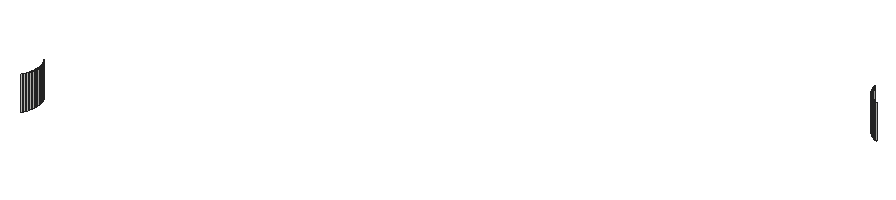
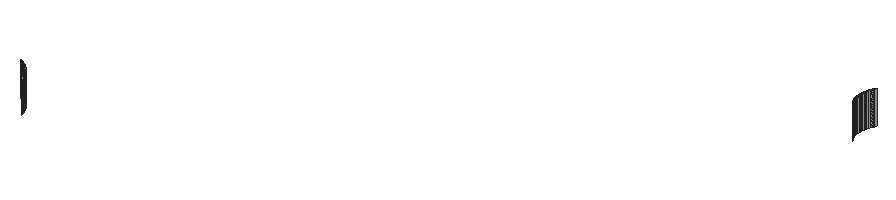
# SketchUp Ruby script. Lengths in inches.
U = 1.inch
M = Sketchup.active_model
def pt(a) = Geom::Point3d.new(a.map { |v| v * U })
def face(e, loops, mat)
  f = e.add_face(loops[0].map { |a| pt(a) })
  loops[1..].each { |l| e.add_face(l.map { |a| pt(a) }).erase! }
  f.material = f.back_material = mat if mat
  f
end
# faces: each face lists its corners as indices into pts; further lists are holes
def faces(e, pts, list, mat = nil) = list.each { |f| face(e, (f[0].is_a?(Array) ? f : [f]).map { |l| l.map { |i| pts[i] } }, mat) }
# xy, xz, yz: faces in a plane at the given z, y or x. An outline is a flat list of corners, or four numbers for a rectangle; further outlines are holes
def ring(l) = l.size == 4 ? [[l[0], l[1]], [l[2], l[1]], [l[2], l[3]], [l[0], l[3]]] : l.each_slice(2).to_a
def flat(e, list, mat, &to3) = list.each { |f| face(e, (f[0].is_a?(Array) ? f : [f]).map { |l| ring(l).map { |u, v| to3.(u, v) } }, mat) }
def xy(e, z, list, mat = nil) = flat(e, list, mat) { |x, y| [x, y, z] }
def xz(e, y, list, mat = nil) = flat(e, list, mat) { |x, z| [x, y, z] }
def yz(e, x, list, mat = nil) = flat(e, list, mat) { |y, z| [x, y, z] }
def lines(e, pts, list) = list.each { |a, b| e.add_line(pt(pts[a]), pt(pts[b])) }
# prism: a flat outline (further loops are holes) pulled along v
def prism(e, loops, v, mat = nil)
  f = face(e, loops, mat); d = Geom::Vector3d.new(v.map { |x| x * U })
  f.pushpull(f.normal.samedirection?(d) ? d.length : -d.length)
end
def box(e, o, s, mat = nil) = prism(e, [[o, [o[0] + s[0], o[1], o[2]], [o[0] + s[0], o[1] + s[1], o[2]], [o[0], o[1] + s[1], o[2]]]], [0, 0, s[2]], mat)
def at(x, y, z, deg = 0) = Geom::Transformation.translation(pt([x, y, z])) * Geom::Transformation.rotation(ORIGIN, Z_AXIS, deg.degrees)
def axes(o, x, y, z) = Geom::Transformation.new([*x, 0, *y, 0, *z, 0, *pt(o).to_a, 1])
def part(name) = M.definitions.add(name)
# library, detail: a bought-in or finely detailed component or shape, given as its bounding box
def library(name, o, s) = part(name).tap { |d| box(d.entities, o, s) }
def detail(e, o, s) = box(e.add_group.entities, o, s)
def put(e, d, t, mat = nil) = e.add_instance(d, t).tap { |i| i.material = mat if mat }
def group(e, t, mat = nil) = e.add_group.tap { |g| g.transformation = t; g.material = mat if mat }.entities
root = M.entities
yz(root,37.5,[[155.77,242,155.85,245],[155.85,242,155.92,245],[155.92,242,156,245],[156,242,156.08,245]])
p = [[37.15,154.65,242],[37.11,154.58,242],[37.11,154.58,245],[37.15,154.65,245],[37.19,154.72,242],[37.19,154.72,245],
  [37.23,154.79,242],[37.23,154.79,245],[37.26,154.86,242],[37.26,154.86,245],[37.29,154.93,242],[37.29,154.93,245],
  [37.32,155,242],[37.32,155,245],[37.35,155.08,242],[37.35,155.08,245],[37.38,155.15,242],[37.38,155.15,245],
  [37.4,155.23,242],[37.4,155.23,245],[37.42,155.3,242],[37.42,155.3,245],[37.44,155.38,242],[37.44,155.38,245],
  [37.46,155.46,242],[37.46,155.46,245],[37.47,155.53,242],[37.47,155.53,245],[37.48,155.61,242],[37.48,155.61,245],
  [37.49,155.6875,242],[37.49,155.6875,245],[37.5,155.77,242],[37.5,155.77,245],[37.49,156.16,242],[37.5,156.08,242],
  [37.5,156.08,245],[37.49,156.16,245],[37.47,156.32,242],[37.48,156.24,242],[37.48,156.24,245],[37.47,156.32,245],
  [37.46,156.39,242],[37.46,156.39,245],[37.44,156.47,242],[37.44,156.47,245],[37.4,156.62,242],[37.42,156.55,242],
  [37.42,156.55,245],[37.4,156.62,245],[37.38,156.7,242],[37.38,156.7,245],[37.35,156.77,242],[37.35,156.77,245],
  [37.29,156.92,242],[37.32,156.84,242],[37.32,156.84,245],[37.29,156.92,245],[37.26,156.99,242],[37.26,156.99,245],
  [37.23,157.06,242],[37.23,157.06,245],[37.15,157.2,242],[37.19,157.13,242],[37.19,157.13,245],[37.15,157.2,245],
  [86.15,188.65,242],[86.08,188.68,242],[86.08,188.68,245],[86.15,188.65,245],[85.9375,188.74,242],[85.87,188.77,242],
  [85.87,188.77,245],[85.9375,188.74,245],[86.01,188.71,242],[86.01,188.71,245],[85.73,188.85,242],[85.66,188.89,242],
  [85.66,188.89,245],[85.73,188.85,245],[85.8,188.81,242],[85.8,188.81,245],[85.59,188.93,242],[85.53,188.98,242],
  [85.53,188.98,245],[85.59,188.93,245],[85.47,189.02,242],[85.41,189.07,242],[85.41,189.07,245],[85.47,189.02,245],
  [85.35,189.125,242],[85.29,189.18,242],[85.29,189.18,245],[85.35,189.125,245],[85.23,189.23,242],[85.18,189.29,242],
  [85.18,189.29,245],[85.23,189.23,245],[85.125,189.35,242],[85.07,189.41,242],[85.07,189.41,245],[85.125,189.35,245],
  [85.02,189.47,242],[85.02,189.47,245],[84.98,189.53,242],[84.93,189.59,242],[84.93,189.59,245],[84.98,189.53,245],
  [84.89,189.66,242],[84.89,189.66,245],[84.85,189.73,242],[84.81,189.8,242],[84.81,189.8,245],[84.85,189.73,245],
  [84.77,189.87,242],[84.77,189.87,245],[84.74,189.9375,242],[84.71,190.01,242],[84.71,190.01,245],[84.74,189.9375,245],
  [84.68,190.08,242],[84.68,190.08,245],[84.65,190.15,242],[84.65,190.15,245],[84.62,190.23,242],[84.6,190.3,242],
  [84.6,190.3,245],[84.62,190.23,245],[84.58,190.38,242],[84.58,190.38,245],[84.56,190.45,242],[84.56,190.45,245]]
faces(root,p,[[0,1,2,3],[4,0,3,5],[6,4,5,7],[8,6,7,9],[10,8,9,11],[12,10,11,13],[14,12,13,15],[16,14,15,17],
  [18,16,17,19],[20,18,19,21],[22,20,21,23],[24,22,23,25],[26,24,25,27],[28,26,27,29],[30,28,29,31],[32,30,31,33],
  [34,35,36,37],[38,39,40,41],[39,34,37,40],[42,38,41,43],[44,42,43,45],[46,47,48,49],[47,44,45,48],[50,46,49,51],
  [52,50,51,53],[54,55,56,57],[55,52,53,56],[58,54,57,59],[60,58,59,61],[62,63,64,65],[63,60,61,64],[66,67,68,69],
  [70,71,72,73],[74,70,73,75],[67,74,75,68],[76,77,78,79],[80,76,79,81],[71,80,81,72],[82,83,84,85],[77,82,85,78],
  [86,87,88,89],[83,86,89,84],[90,91,92,93],[87,90,93,88],[94,95,96,97],[91,94,97,92],[98,99,100,101],[95,98,101,96],
  [99,102,103,100],[104,105,106,107],[102,104,107,103],[105,108,109,106],[110,111,112,113],[108,110,113,109],[111,114,115,112],[116,117,118,119],
  [114,116,119,115],[117,120,121,118],[120,122,123,121],[124,125,126,127],[122,124,127,123],[125,128,129,126],[128,130,131,129]])
